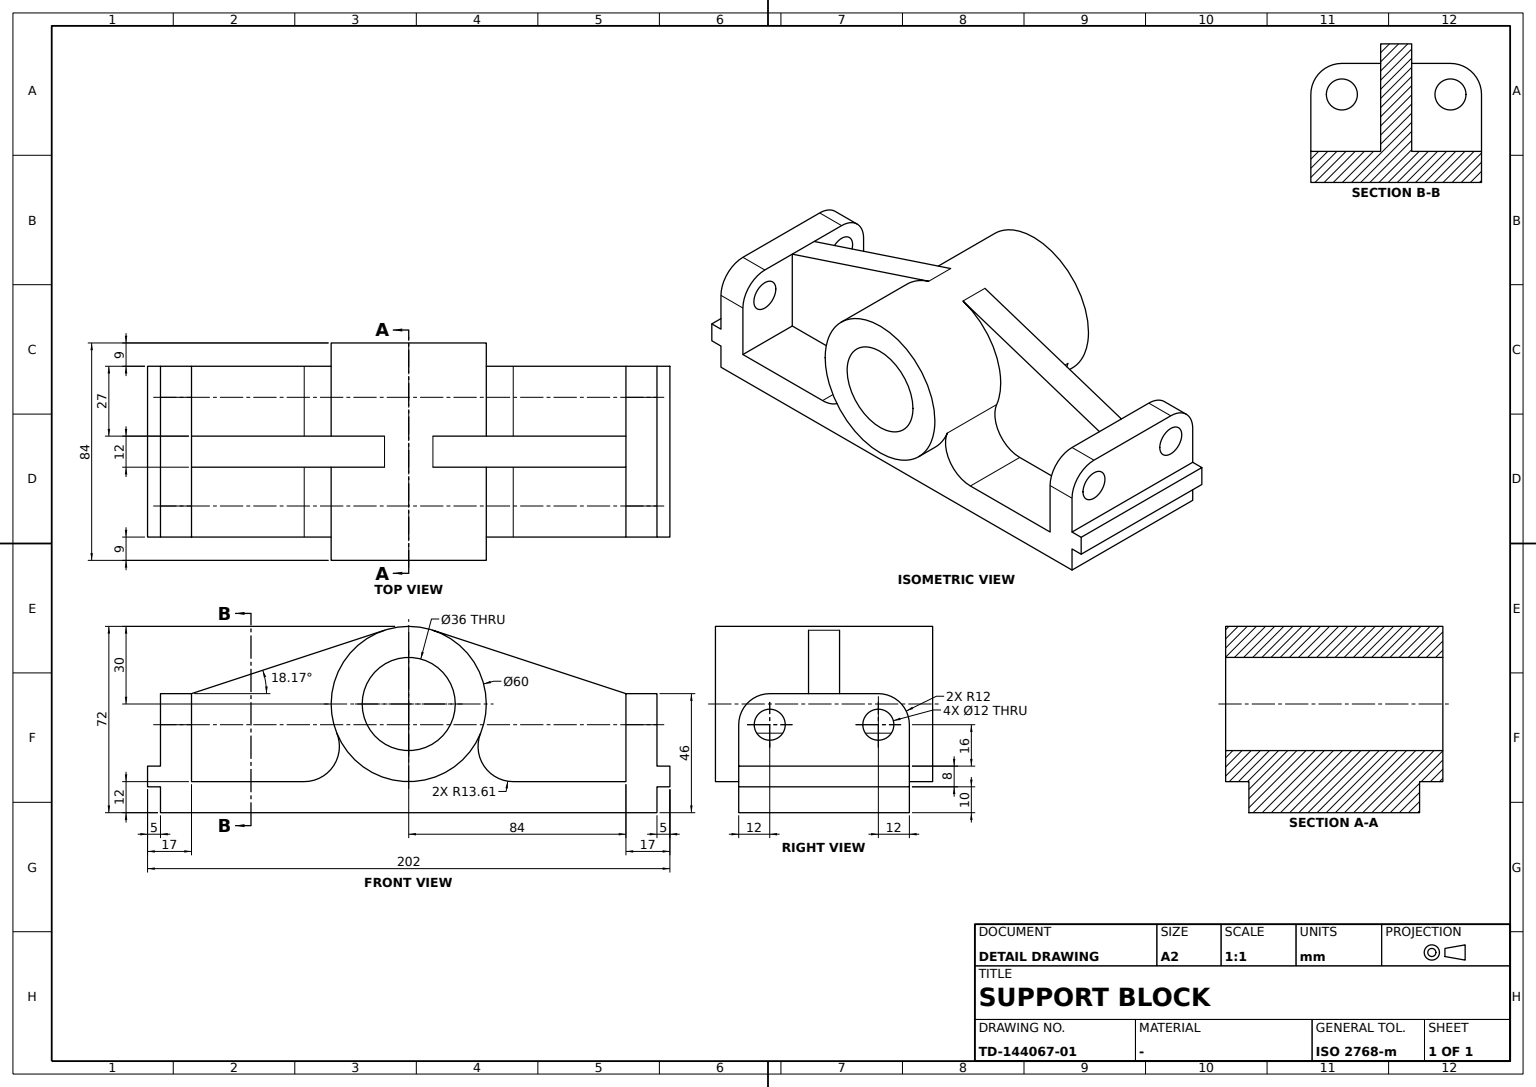
solid
v1 (-33,101,-32)
v2 (-33,101,-24)
e1 v1 v2 LINE
v3 (33,101,-24)
e2 v2 v3 LINE
v4 (33,101,-32)
e3 v4 v3 LINE
e4 v1 v4 LINE
face PLANE(AX(P(0,101,-32),D(0,1,0),D(0,0,1))) [e1 e2 -e3 -e4]
v5 (27,-84,-8)
v6 (15,-84,-8)
e5 v5 v6 CIRCLE(AX(P(21,-84,-8),D(0,-1,0),D(0,0,-1)),6)
v7 (27,-96,-8)
e6 v7 v5 LINE
v8 (15,-96,-8)
e7 v8 v7 CIRCLE(AX(P(21,-96,-8),D(0,1,0),D(0,0,1)),6)
e8 v8 v6 LINE
face CYL(AX(P(21,-3.1600000015,-8),D(0,-1,0),D(-1,0,0)),6) rev [-e5 -e6 -e7 e8]
e9 v6 v5 CIRCLE(AX(P(21,-84,-8),D(0,-1,0),D(0,0,-1)),6)
v9 (6,-84,4)
v10 (21,-84,4)
e10 v9 v10 LINE
v11 (33,-84,-8)
e11 v11 v10 CIRCLE(AX(P(21,-84,-8),D(0,-1,0),D(0,0,-1)),12)
v12 (33,-84,-30)
e12 v12 v11 LINE
v13 (6,-84,-30)
e13 v13 v12 LINE
e14 v9 v13 LINE
face PLANE(AX(P(0,-84,4),D(0,-1,0),D(0,0,-1))) rev [e9 e5] [e10 -e11 -e12 -e13 -e14]
v14 (-33,-26.8039236423,-16.3878242478)
v15 (-33,-40.4160993944,-30)
e15 v14 v15 CIRCLE(AX(P(-33,-40.4160993944,-16.3878242478),D(-1,0,0),D(0,1,0)),13.6121757522)
v16 (-6,-40.4160993944,-30)
e16 v15 v16 LINE
v17 (-6,-26.8039236423,-16.3878242478)
e17 v16 v17 CIRCLE(AX(P(-6,-40.4160993944,-16.3878242478),D(1,0,0),D(0,1,0)),13.6121757522)
e18 v17 v14 LINE
face CYL(AX(P(0,-40.4160993944,-16.3878242478),D(-1,0,0),D(0,1,0)),13.6121757522) rev [e15 e16 e17 e18]
v18 (-6,9.3569783252,28.5034551699)
v19 (6,9.3569783252,28.5034551699)
e19 v18 v19 LINE
v20 (6,84,4)
e20 v19 v20 LINE
v21 (-6,84,4)
e21 v21 v20 LINE
e22 v18 v21 LINE
face PLANE(AX(P(0,9.3569783252,28.5034551699),D(0,0.3118992775,0.9501151723),D(0,-0.9501151723,0.3118992775))) [e19 e20 -e21 -e22]
v22 (-33,-101,-24)
v23 (-33,-101,-32)
e23 v22 v23 LINE
v24 (33,-101,-32)
e24 v23 v24 LINE
v25 (33,-101,-24)
e25 v25 v24 LINE
e26 v22 v25 LINE
face PLANE(AX(P(0,-101,-32),D(0,1,0),D(0,0,1))) rev [e23 e24 -e25 -e26]
v26 (-6,-30,0)
v27 (-42,-30,0)
e27 v26 v27 LINE
v28 (-6,-9.3569783252,28.5034551699)
e28 v28 v26 CIRCLE(AX(P(-6,0,0),D(1,0,0),D(0,1,0)),30)
v29 (6,-9.3569783252,28.5034551699)
e29 v28 v29 LINE
v30 (6,-30,0)
e30 v29 v30 CIRCLE(AX(P(6,0,0),D(1,0,0),D(0,1,0)),30)
v31 (42,-30,0)
e31 v31 v30 LINE
v32 (42,30,0)
e32 v32 v31 CIRCLE(AX(P(42,0,0),D(1,0,0),D(0,1,0)),30)
v33 (6,30,0)
e33 v32 v33 LINE
e34 v19 v33 CIRCLE(AX(P(6,0,0),D(-1,0,0),D(0,1,0)),30)
v34 (-6,30,0)
e35 v18 v34 CIRCLE(AX(P(-6,0,0),D(-1,0,0),D(0,1,0)),30)
v35 (-42,30,0)
e36 v34 v35 LINE
e37 v35 v27 CIRCLE(AX(P(-42,0,0),D(1,0,0),D(0,1,0)),30)
face CYL(AX(P(0,0,0),D(-1,0,0),D(0,1,0)),30) [-e27 -e28 e29 e30 -e31 -e32 e33 -e34 -e19 e35 e36 e37]
v36 (-6,27.8014788513,-11.2728777906)
e38 v34 v36 CIRCLE(AX(P(-6,0,0),D(-1,0,0),D(0,1,0)),30)
v37 (-33,27.8014788513,-11.2728777906)
e39 v37 v36 LINE
v38 (-42,27.8014788513,-11.2728777906)
e40 v38 v37 LINE
e41 v38 v35 CIRCLE(AX(P(-42,0,0),D(1,0,0),D(0,1,0)),30)
face CYL(AX(P(0,0,0),D(-1,0,0),D(0,1,0)),30) [-e36 e38 -e39 -e40 e41]
v39 (-27,96,-8)
v40 (-27,84,-8)
e42 v39 v40 LINE
v41 (-15,84,-8)
e43 v40 v41 CIRCLE(AX(P(-21,84,-8),D(0,-1,0),D(0,0,-1)),6)
v42 (-15,96,-8)
e44 v42 v41 LINE
e45 v42 v39 CIRCLE(AX(P(-21,96,-8),D(0,1,0),D(-1,0,0)),6)
face CYL(AX(P(-21,-3.1600000015,-8),D(0,-1,0),D(-1,0,0)),6) rev [e42 e43 -e44 e45]
v43 (27,96,-8)
v44 (27,84,-8)
e46 v43 v44 LINE
v45 (15,84,-8)
e47 v44 v45 CIRCLE(AX(P(21,84,-8),D(0,-1,0),D(0,0,-1)),6)
v46 (15,96,-8)
e48 v46 v45 LINE
e49 v46 v43 CIRCLE(AX(P(21,96,-8),D(0,1,0),D(-1,0,0)),6)
face CYL(AX(P(21,-3.1600000015,-8),D(0,-1,0),D(-1,0,0)),6) rev [e46 e47 -e48 e49]
e50 v7 v8 CIRCLE(AX(P(21,-96,-8),D(0,1,0),D(0,0,1)),6)
face CYL(AX(P(21,-3.1600000015,-8),D(0,-1,0),D(-1,0,0)),6) rev [-e9 -e8 -e50 e6]
v47 (-33,-96,-32)
e51 v23 v47 LINE
v48 (33,-96,-32)
e52 v47 v48 LINE
e53 v24 v48 LINE
face PLANE(AX(P(0,-96,-32),D(0,0,1),D(0,-1,0))) rev [e51 e52 -e53 -e24]
v49 (-33,96,-24)
v50 (33,96,-24)
e54 v49 v50 LINE
e55 v3 v50 LINE
e56 v2 v49 LINE
face PLANE(AX(P(0,-101,-24),D(0,0,-1),D(0,1,0))) rev [e54 -e55 -e2 e56]
e57 v39 v42 CIRCLE(AX(P(-21,96,-8),D(0,1,0),D(-1,0,0)),6)
e58 v41 v40 CIRCLE(AX(P(-21,84,-8),D(0,-1,0),D(0,0,-1)),6)
face CYL(AX(P(-21,-3.1600000015,-8),D(0,-1,0),D(-1,0,0)),6) rev [e57 e44 e58 -e42]
v51 (6,84,-30)
v52 (33,84,-30)
e59 v51 v52 LINE
v53 (6,40.4160993944,-30)
e60 v51 v53 LINE
v54 (33,40.4160993944,-30)
e61 v53 v54 LINE
e62 v52 v54 LINE
face PLANE(AX(P(0,-84,-30),D(0,0,-1),D(0,1,0))) rev [-e59 e60 e61 -e62]
v55 (-15,-96,-8)
v56 (-27,-96,-8)
e63 v55 v56 CIRCLE(AX(P(-21,-96,-8),D(0,1,0),D(0,0,1)),6)
e64 v56 v55 CIRCLE(AX(P(-21,-96,-8),D(0,1,0),D(0,0,1)),6)
v57 (21,-96,4)
v58 (33,-96,-8)
e65 v57 v58 CIRCLE(AX(P(21,-96,-8),D(0,1,0),D(0,0,1)),12)
v59 (-21,-96,4)
e66 v59 v57 LINE
v60 (-33,-96,-8)
e67 v60 v59 CIRCLE(AX(P(-21,-96,-8),D(0,1,0),D(0,0,1)),12)
v61 (-33,-96,-24)
e68 v60 v61 LINE
v62 (33,-96,-24)
e69 v61 v62 LINE
e70 v58 v62 LINE
face PLANE(AX(P(0,-96,-24),D(0,1,0),D(0,0,1))) rev [e63 e64] [-e65 -e66 -e67 e68 e69 -e70] [e50 e7]
v63 (-33,96,-8)
e71 v49 v63 LINE
v64 (-21,96,4)
e72 v64 v63 CIRCLE(AX(P(-21,96,-8),D(0,-1,0),D(0,0,1)),12)
v65 (21,96,4)
e73 v64 v65 LINE
v66 (33,96,-8)
e74 v66 v65 CIRCLE(AX(P(21,96,-8),D(0,-1,0),D(0,0,1)),12)
e75 v50 v66 LINE
e76 v43 v46 CIRCLE(AX(P(21,96,-8),D(0,1,0),D(-1,0,0)),6)
face PLANE(AX(P(0,96,-42),D(0,1,0),D(0,0,1))) [e71 -e72 e73 -e74 -e75 -e54] [-e57 -e45] [-e49 -e76]
v67 (33,-27.8014788513,-11.2728777906)
v68 (42,-27.8014788513,-11.2728777906)
e77 v67 v68 LINE
v69 (33,27.8014788513,-11.2728777906)
e78 v67 v69 CIRCLE(AX(P(33,0,0),D(1,0,0),D(0,1,0)),30)
v70 (42,27.8014788513,-11.2728777906)
e79 v69 v70 LINE
e80 v68 v70 CIRCLE(AX(P(42,0,0),D(1,0,0),D(0,1,0)),30)
face CYL(AX(P(0,0,0),D(-1,0,0),D(0,1,0)),30) [-e77 e78 e79 -e80]
v71 (33,84,-8)
e81 v66 v71 LINE
v72 (21,84,4)
e82 v65 v72 LINE
e83 v71 v72 CIRCLE(AX(P(21,84,-8),D(0,-1,0),D(0,0,-1)),12)
face CYL(AX(P(21,0,-8),D(0,1,0),D(0,0,1)),12) [-e81 e74 e82 -e83]
v73 (-33,84,-8)
e84 v63 v73 LINE
v74 (-21,84,4)
e85 v73 v74 CIRCLE(AX(P(-21,84,-8),D(0,1,0),D(0,0,-1)),12)
e86 v64 v74 LINE
face CYL(AX(P(-21,0,-8),D(0,1,0),D(-1,0,0)),12) [e84 e85 -e86 e72]
v75 (6,27.8014788513,-11.2728777906)
e87 v53 v75 CIRCLE(AX(P(6,40.4160993944,-16.3878242478),D(-1,0,0),D(0,1,0)),13.6121757522)
e88 v75 v69 LINE
e89 v54 v69 CIRCLE(AX(P(33,40.4160993944,-16.3878242478),D(-1,0,0),D(0,1,0)),13.6121757522)
face CYL(AX(P(0,40.4160993944,-16.3878242478),D(-1,0,0),D(0,1,0)),13.6121757522) rev [-e61 e87 e88 -e89]
e90 v61 v22 LINE
e91 v62 v25 LINE
face PLANE(AX(P(0,-101,-24),D(0,0,-1),D(0,1,0))) rev [e90 e26 -e91 -e69]
v76 (6,-40.4160993944,-30)
v77 (6,-26.8039236423,-16.3878242478)
e92 v76 v77 CIRCLE(AX(P(6,-40.4160993944,-16.3878242478),D(1,0,0),D(0,1,0)),13.6121757522)
v78 (33,-40.4160993944,-30)
e93 v76 v78 LINE
v79 (33,-26.8039236423,-16.3878242478)
e94 v79 v78 CIRCLE(AX(P(33,-40.4160993944,-16.3878242478),D(-1,0,0),D(0,1,0)),13.6121757522)
e95 v79 v77 LINE
face CYL(AX(P(0,-40.4160993944,-16.3878242478),D(-1,0,0),D(0,1,0)),13.6121757522) rev [-e92 e93 -e94 e95]
v80 (-33,96,-42)
v81 (33,96,-42)
e96 v80 v81 LINE
v82 (33,-96,-42)
e97 v82 v81 LINE
v83 (-33,-96,-42)
e98 v83 v82 LINE
e99 v83 v80 LINE
face PLANE(AX(P(0,96,-42),D(0,0,1),D(0,-1,0))) rev [e96 -e97 -e98 e99]
v84 (-42,-27.8014788513,-11.2728777906)
e100 v84 v38 CIRCLE(AX(P(-42,0,0),D(1,0,0),D(0,1,0)),30)
v85 (-33,-27.8014788513,-11.2728777906)
e101 v85 v37 CIRCLE(AX(P(-33,0,0),D(1,0,0),D(0,1,0)),30)
e102 v84 v85 LINE
face CYL(AX(P(0,0,0),D(-1,0,0),D(0,1,0)),30) [e100 e40 -e101 -e102]
e103 v27 v84 CIRCLE(AX(P(-42,0,0),D(1,0,0),D(0,1,0)),30)
v86 (-6,-27.8014788513,-11.2728777906)
e104 v85 v86 LINE
e105 v26 v86 CIRCLE(AX(P(-6,0,0),D(1,0,0),D(0,1,0)),30)
face CYL(AX(P(0,0,0),D(-1,0,0),D(0,1,0)),30) [e27 e103 e102 e104 -e105]
e106 v31 v68 CIRCLE(AX(P(42,0,0),D(1,0,0),D(0,1,0)),30)
e107 v70 v32 CIRCLE(AX(P(42,0,0),D(1,0,0),D(0,1,0)),30)
v87 (42,18,0)
v88 (42,-18,0)
e108 v87 v88 CIRCLE(AX(P(42,0,0),D(1,0,0),D(0,1,0)),18)
e109 v88 v87 CIRCLE(AX(P(42,0,0),D(1,0,0),D(0,1,0)),18)
face PLANE(AX(P(42,0,0),D(1,0,0),D(0,1,0))) [e106 e80 e107 e32] [-e108 -e109]
e110 v74 v21 LINE
e111 v20 v72 LINE
face PLANE(AX(P(0,-96,4),D(0,0,-1),D(0,1,0))) rev [-e73 e86 e110 e21 e111 -e82]
v89 (-33,40.4160993944,-30)
e112 v89 v37 CIRCLE(AX(P(-33,40.4160993944,-16.3878242478),D(-1,0,0),D(0,1,0)),13.6121757522)
v90 (-6,40.4160993944,-30)
e113 v90 v36 CIRCLE(AX(P(-6,40.4160993944,-16.3878242478),D(-1,0,0),D(0,1,0)),13.6121757522)
e114 v89 v90 LINE
face CYL(AX(P(0,40.4160993944,-16.3878242478),D(-1,0,0),D(0,1,0)),13.6121757522) rev [e112 e39 -e113 -e114]
v91 (-21,-84,4)
e115 v91 v59 LINE
v92 (-33,-84,-8)
e116 v91 v92 CIRCLE(AX(P(-21,-84,-8),D(0,-1,0),D(0,0,-1)),12)
e117 v92 v60 LINE
face CYL(AX(P(-21,0,-8),D(0,-1,0),D(-1,0,0)),12) [e67 -e115 e116 e117]
v93 (-6,-84,4)
e118 v28 v93 LINE
e119 v93 v9 LINE
e120 v29 v9 LINE
face PLANE(AX(P(0,-9.3569783252,28.5034551699),D(0,0.3118992775,-0.9501151723),D(0,0.9501151723,0.3118992775))) rev [e118 e119 -e120 -e29]
v94 (-33,96,-32)
e121 v80 v94 LINE
v95 (33,96,-32)
e122 v94 v95 LINE
e123 v81 v95 LINE
face PLANE(AX(P(0,96,-42),D(0,1,0),D(0,0,1))) [-e96 e121 e122 -e123]
v96 (-42,-18,0)
e124 v96 v88 LINE
v97 (-42,18,0)
e125 v97 v96 CIRCLE(AX(P(-42,0,0),D(1,0,0),D(0,1,0)),18)
e126 v97 v87 LINE
face CYL(AX(P(0,0,0),D(-1,0,0),D(0,1,0)),18) rev [e108 -e124 -e125 e126]
e127 v33 v75 CIRCLE(AX(P(6,0,0),D(-1,0,0),D(0,1,0)),30)
face CYL(AX(P(0,0,0),D(-1,0,0),D(0,1,0)),30) [-e79 -e88 -e127 -e33 -e107]
v98 (-33,84,-30)
e128 v73 v98 LINE
v99 (-6,84,-30)
e129 v98 v99 LINE
e130 v21 v99 LINE
face PLANE(AX(P(0,84,4),D(0,-1,0),D(0,0,-1))) [-e43 -e58] [-e110 -e85 e128 e129 -e130]
e131 v78 v12 LINE
e132 v13 v76 LINE
face PLANE(AX(P(0,-84,-30),D(0,0,-1),D(0,1,0))) rev [e13 -e131 -e93 -e132]
e133 v71 v52 LINE
e134 v20 v51 LINE
e135 v45 v44 CIRCLE(AX(P(21,84,-8),D(0,-1,0),D(0,0,-1)),6)
face PLANE(AX(P(0,84,4),D(0,-1,0),D(0,0,-1))) [e59 -e133 e83 -e111 e134] [-e135 -e47]
e136 v10 v57 LINE
e137 v11 v58 LINE
face CYL(AX(P(21,0,-8),D(0,-1,0),D(0,0,1)),12) [e136 e65 -e137 e11]
e138 v99 v90 LINE
face PLANE(AX(P(-6,0,0),D(1,0,0),D(0,1,0))) rev [e130 e138 e113 -e38 -e35 e22]
e139 v17 v86 CIRCLE(AX(P(-6,-40.4160993944,-16.3878242478),D(1,0,0),D(0,1,0)),13.6121757522)
v100 (-6,-84,-30)
e140 v100 v16 LINE
e141 v93 v100 LINE
face PLANE(AX(P(-6,0,0),D(1,0,0),D(0,1,0))) rev [e28 e105 -e139 -e17 -e140 -e141 -e118]
e142 v94 v1 LINE
e143 v47 v83 LINE
v101 (-33,-84,-30)
e144 v101 v92 LINE
e145 v15 v101 LINE
e146 v85 v14 CIRCLE(AX(P(-33,-40.4160993944,-16.3878242478),D(-1,0,0),D(0,1,0)),13.6121757522)
e147 v98 v89 LINE
face PLANE(AX(P(-33,0,0),D(1,0,0),D(0,1,0))) rev [-e142 -e121 -e99 -e143 -e51 -e23 -e90 -e68 -e117 -e144 -e145 -e15 -e146 e101 -e112 -e147 -e128 -e84 -e71 -e56 -e1]
v102 (6,-27.8014788513,-11.2728777906)
e148 v30 v102 CIRCLE(AX(P(6,0,0),D(1,0,0),D(0,1,0)),30)
e149 v102 v67 LINE
face CYL(AX(P(0,0,0),D(-1,0,0),D(0,1,0)),30) [e77 -e106 e31 e148 e149]
e150 v67 v79 CIRCLE(AX(P(33,-40.4160993944,-16.3878242478),D(-1,0,0),D(0,1,0)),13.6121757522)
e151 v48 v82 LINE
e152 v95 v4 LINE
face PLANE(AX(P(33,0,0),D(1,0,0),D(0,1,0))) [e133 e62 e89 -e78 e150 e94 e131 e12 e137 e70 e91 e25 e53 e151 e97 e123 e152 e3 e55 e75 e81]
face PLANE(AX(P(0,-96,-32),D(0,0,1),D(0,-1,0))) rev [-e122 e142 e4 -e152]
e153 v96 v97 CIRCLE(AX(P(-42,0,0),D(1,0,0),D(0,1,0)),18)
face PLANE(AX(P(-42,0,0),D(1,0,0),D(0,1,0))) rev [e125 e153] [-e41 -e100 -e103 -e37]
face PLANE(AX(P(6,0,0),D(1,0,0),D(0,1,0))) [-e87 -e60 -e134 -e20 e34 e127]
e154 v77 v102 CIRCLE(AX(P(6,-40.4160993944,-16.3878242478),D(1,0,0),D(0,1,0)),13.6121757522)
face PLANE(AX(P(6,0,0),D(1,0,0),D(0,1,0))) [-e148 -e30 e120 e14 e132 e92 e154]
v103 (-27,-84,-8)
e155 v56 v103 LINE
v104 (-15,-84,-8)
e156 v104 v103 CIRCLE(AX(P(-21,-84,-8),D(0,-1,0),D(0,0,-1)),6)
e157 v55 v104 LINE
face CYL(AX(P(-21,-3.1600000015,-8),D(0,-1,0),D(-1,0,0)),6) rev [-e64 e155 -e156 -e157]
e158 v91 v93 LINE
face PLANE(AX(P(0,-96,4),D(0,0,-1),D(0,1,0))) rev [-e158 e115 e66 -e136 -e10 -e119]
e159 v101 v100 LINE
face PLANE(AX(P(0,-84,-30),D(0,0,-1),D(0,1,0))) rev [e140 -e16 e145 e159]
e160 v103 v104 CIRCLE(AX(P(-21,-84,-8),D(0,-1,0),D(0,0,-1)),6)
face PLANE(AX(P(0,-84,4),D(0,-1,0),D(0,0,-1))) rev [e156 e160] [e141 -e159 e144 -e116 e158]
face PLANE(AX(P(0,-84,-30),D(0,0,-1),D(0,1,0))) rev [-e129 e147 e114 -e138]
face CYL(AX(P(21,-3.1600000015,-8),D(0,-1,0),D(-1,0,0)),6) rev [e48 e135 -e46 e76]
face CYL(AX(P(0,0,0),D(-1,0,0),D(0,1,0)),18) rev [e124 e109 -e126 -e153]
face CYL(AX(P(0,-40.4160993944,-16.3878242478),D(-1,0,0),D(0,1,0)),13.6121757522) rev [-e18 e139 -e104 e146]
face CYL(AX(P(-21,-3.1600000015,-8),D(0,-1,0),D(-1,0,0)),6) rev [-e160 -e155 -e63 e157]
face PLANE(AX(P(0,-96,-24),D(0,1,0),D(0,0,1))) rev [e143 e98 -e151 -e52]
face CYL(AX(P(0,-40.4160993944,-16.3878242478),D(-1,0,0),D(0,1,0)),13.6121757522) rev [-e149 -e154 -e95 -e150]
